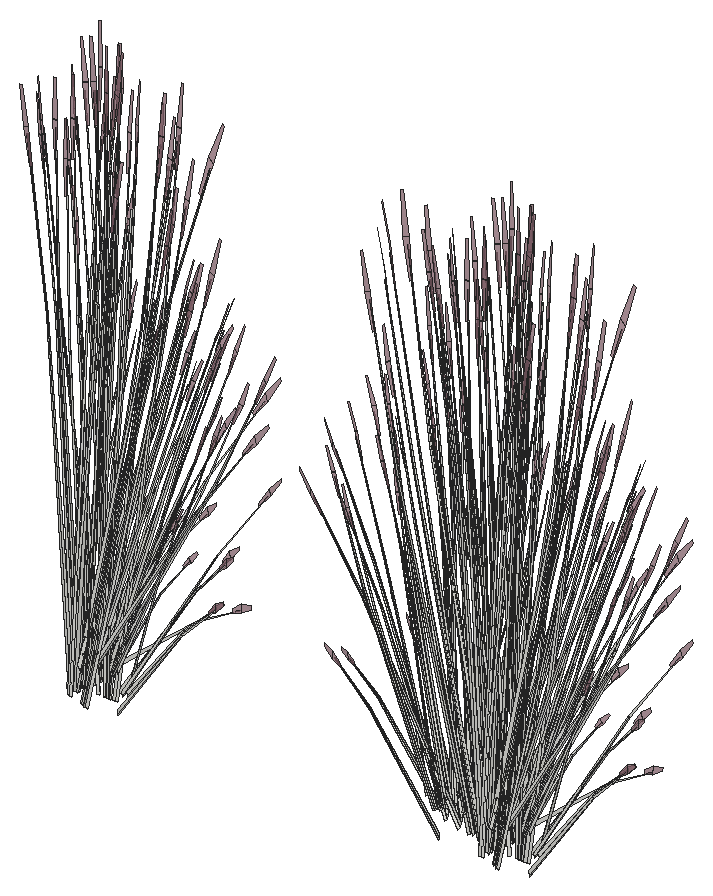
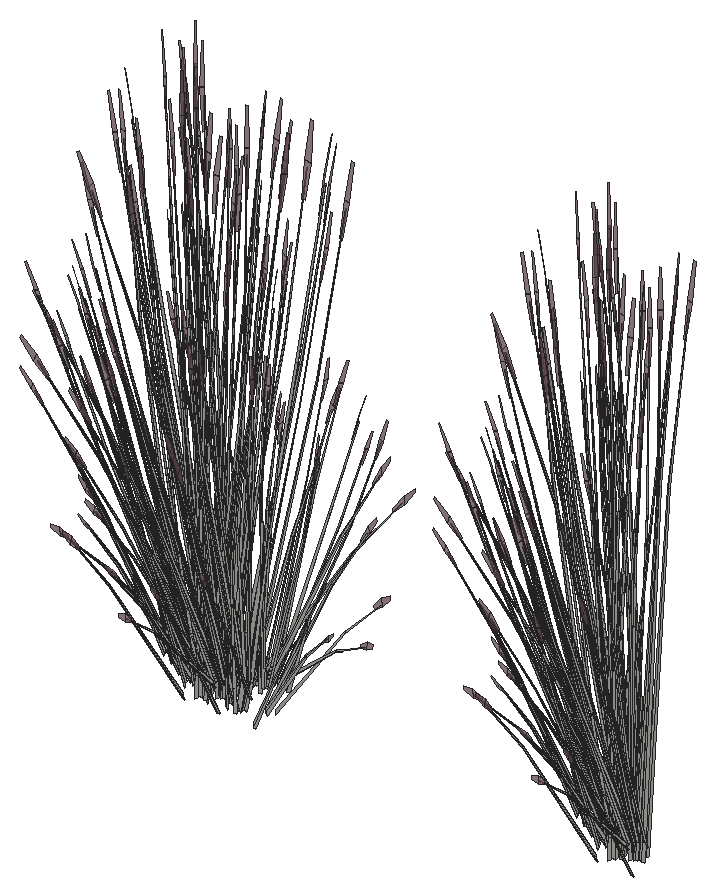
# SketchUp Ruby script. Lengths in inches.
U = 1.inch
M = Sketchup.active_model
def pt(a) = Geom::Point3d.new(a.map { |v| v * U })
def face(e, loops, mat)
  f = e.add_face(loops[0].map { |a| pt(a) })
  loops[1..].each { |l| e.add_face(l.map { |a| pt(a) }).erase! }
  f.material = f.back_material = mat if mat
  f
end
# faces: each face lists its corners as indices into pts; further lists are holes
def faces(e, pts, list, mat = nil) = list.each { |f| face(e, (f[0].is_a?(Array) ? f : [f]).map { |l| l.map { |i| pts[i] } }, mat) }
# xy, xz, yz: faces in a plane at the given z, y or x. An outline is a flat list of corners, or four numbers for a rectangle; further outlines are holes
def ring(l) = l.size == 4 ? [[l[0], l[1]], [l[2], l[1]], [l[2], l[3]], [l[0], l[3]]] : l.each_slice(2).to_a
def flat(e, list, mat, &to3) = list.each { |f| face(e, (f[0].is_a?(Array) ? f : [f]).map { |l| ring(l).map { |u, v| to3.(u, v) } }, mat) }
def xy(e, z, list, mat = nil) = flat(e, list, mat) { |x, y| [x, y, z] }
def xz(e, y, list, mat = nil) = flat(e, list, mat) { |x, z| [x, y, z] }
def yz(e, x, list, mat = nil) = flat(e, list, mat) { |y, z| [x, y, z] }
def lines(e, pts, list) = list.each { |a, b| e.add_line(pt(pts[a]), pt(pts[b])) }
# prism: a flat outline (further loops are holes) pulled along v
def prism(e, loops, v, mat = nil)
  f = face(e, loops, mat); d = Geom::Vector3d.new(v.map { |x| x * U })
  f.pushpull(f.normal.samedirection?(d) ? d.length : -d.length)
end
def box(e, o, s, mat = nil) = prism(e, [[o, [o[0] + s[0], o[1], o[2]], [o[0] + s[0], o[1] + s[1], o[2]], [o[0], o[1] + s[1], o[2]]]], [0, 0, s[2]], mat)
def at(x, y, z, deg = 0) = Geom::Transformation.translation(pt([x, y, z])) * Geom::Transformation.rotation(ORIGIN, Z_AXIS, deg.degrees)
def axes(o, x, y, z) = Geom::Transformation.new([*x, 0, *y, 0, *z, 0, *pt(o).to_a, 1])
def part(name) = M.definitions.add(name)
# library, detail: a bought-in or finely detailed component or shape, given as its bounding box
def library(name, o, s) = part(name).tap { |d| box(d.entities, o, s) }
def detail(e, o, s) = box(e.add_group.entities, o, s)
def put(e, d, t, mat = nil) = e.add_instance(d, t).tap { |i| i.material = mat if mat }
def group(e, t, mat = nil) = e.add_group.tap { |g| g.transformation = t; g.material = mat if mat }.entities
root = M.entities
M.materials.add("LightPink_Translucent").color = [144, 107, 117]
M.materials["LightPink_Translucent"].alpha = 0.75
c1 = part("blade")
p = [[2.15,0.21,22],[0,0.17,0],[0.09,0.45,0],[2.18,0.31,22],[2.29,0.31,22],[0.38,0.45,0],
  [2.48,0.24,33],[2.49,0.24,33],[2.48,0.22,33]]
faces(c1.entities,p,[[0,1,2,3],[4,5,2,3],[6,3,4,7],[8,0,3,6]])
c2 = part("seeds")
p = [[0.3,-0.1,1.38],[-0.01,-0.03,1.59],[-0.01,-0.03,0.03],[0.14,-0.07,-0.07],[0.29,-0.03,3],[0.15,0.01,3.11]]
faces(c2.entities,p,[[0,1,2,3],[1,0,4,5]],"LightPink_Translucent")
c3 = part("blade with seeds")
put(c3.entities,c1,at(0,0,0))
put(c3.entities,c2,axes([2.4,0.25,30.99],[1.5799,-0.05474,1.17369],[-0.12525,1.92788,0.29478],[-0.07173,-0.02425,1.56792]))
put(root,c3,axes([817.6,482.08,3.9375],[-0.01125,-0.12549,0.85688],[0.48751,0.08325,0.06928],[-0.03015,0.17883,0.36631]))
put(root,c3,axes([818.01,481.54,3.18],[0.58084,0.06889,0.22877],[-0.11821,0.38906,0.08977],[-0.08488,-0.03757,0.79428]))
put(root,c3,axes([817.7,482.16,3.24],[0.49383,-0.08678,0.08821],[0.12194,0.32295,0.17543],[-0.04404,-0.04705,0.80203]))
put(root,c3,axes([818.33,482.21,3.1],[-0.4633,-0.14679,0],[0.22297,-0.30501,0],[0,0,0.81353]))
put(root,c3,axes([819.41,482.58,3.1875],[0.28732,0.32763,0],[-0.4807,0.18271,-0.25804],[-0.10948,0.04161,0.81856]))
put(root,c3,axes([817.94,482.72,4.53],[-0.45283,-0.08548,0.26641],[0.15485,-0.28101,0.21967],[0.02721,0.11051,0.55128]))
put(root,c3,axes([817.82,482.74,4.37],[-0.33863,0.11112,0.03215],[-0.16575,-0.20263,0.2531],[0.0327,0.08932,0.38595]))
put(root,c3,axes([819.17,482.18,3.24],[0.13276,-0.32494,0.08821],[0.4858,0.09195,0.17543],[-0.08392,0.00158,0.80203]))
put(root,c3,axes([818.94,481.75,3.31],[0.33952,0.19644,0.0724],[-0.2832,0.22163,-0.20674],[-0.07883,0.02996,0.63372]))
put(root,c3,axes([818.94,481.6,3.36],[0.49904,-0.02018,0.2237],[0.04513,0.33504,-0.10766],[-0.08934,0.03396,0.71822]))
put(root,c3,axes([819.06,482.375,3.17],[0.57533,0.10627,0.15378],[-0.14394,0.37986,-0.18246],[-0.09522,0.04754,0.82443]))
put(root,c3,axes([819.3,482.35,3.24],[0.4301,-0.16348,0.24825],[0.25708,0.29314,0],[-0.09796,0.03723,0.78752]))
put(root,c3,axes([818.44,482.09,3.1],[-0.14994,-0.28188,0],[0.42817,-0.09871,0],[0,0,0.77185]))
put(root,c3,axes([817.89,482.68,2.75],[0.07437,-0.01779,0.88171],[0.44738,0.09793,-0.1347],[0.01308,0.11037,0.15018]))
put(root,c3,axes([817.99,482.78,4.26],[-0.13855,0.25143,-0.17707],[-0.4042,-0.07334,0.2286],[0.03706,0.10123,0.4374]))
put(root,c3,axes([819.04,481.53,3.11],[-0.22297,0.29461,-0.2237],[-0.4633,-0.14179,0.10766],[0,0.06791,0.71822]))
put(root,c3,axes([817.71,483.23,4.36],[0.05825,0.05265,0.87472],[0.47011,0.02068,-0.13834],[0.04727,0.11612,0.07015]))
put(root,c3,axes([819.93,481.35,3.24],[-0.36107,-0.23816,0.08821],[0.36387,-0.231,0.17543],[-0.03988,0.04864,0.80203]))
put(root,c3,axes([818.97,481.36,3.15],[0,0.37813,-0.02818],[-0.57465,0,0],[0,0.01188,0.89684]))
put(root,c3,axes([817.95,482.51,4.53],[0.13855,-0.25143,0.17707],[0.4042,0.07334,-0.2286],[0.03706,0.10123,0.4374]))
put(root,c3,axes([818.69,482.1,3.15],[0.1998,0.37562,-0.03006],[-0.5709,0.13162,0],[0.00698,0.01312,0.86086]))
put(root,c3,axes([818.04,482.55,4.49],[0.21934,0.26585,-0.35523],[-0.45151,0.14816,0.04287],[0.05129,0.12845,0.5025]))
put(root,c3,axes([820.34,481.6,3.1],[-0.57436,-0.00261,-0.02488],[0,-0.36542,0.24971],[-0.01805,0.08319,0.79176]))
put(root,c3,axes([819.21,480.5,3.24],[-0.49383,0.08678,0.08821],[-0.12194,-0.32295,0.17543],[0.04404,0.04705,0.80203]))
put(root,c3,axes([818.49,483.41,4.82],[0.31757,-0.18757,-0.03244],[0.29098,0.20543,-0.14708],[0.02049,0.05821,0.48512]))
put(root,c3,axes([819.06,481.44,3.11],[0.32079,0.21119,0],[-0.32079,0.21119,0],[0,0,0.84633]))
put(root,c3,axes([819.05,481.19,3.36],[0.22297,-0.29461,0.2237],[0.4633,0.14179,-0.10766],[0,0.06791,0.71822]))
put(root,c3,axes([818.86,482.22,3.1],[0.4633,0.14679,0],[-0.22297,0.30501,0],[0,0,0.87477]))
put(root,c3,axes([818.2,482.61,4.34],[0.45175,0.08196,-0.25549],[-0.15485,0.28101,-0.1979],[0.04142,0.11314,0.48886]))
put(root,c3,axes([817.8125,482.62,4.52],[0.44971,-0.15222,-0.0608],[0.221,0.27017,-0.33747],[0.05933,0.11385,0.51278]))
put(root,c3,axes([818.9,481.125,3.19],[-0.58084,-0.06889,0.24599],[0.11821,-0.38906,0.09653],[0.08488,0.03757,0.85407]))
put(root,c3,axes([820.22,481.66,3.01],[-0.32079,0.20399,-0.15489],[-0.32079,-0.20399,0.15489],[0,0.06571,0.69487]))
put(root,c3,axes([819.31,481.62,3.05],[0.16851,0.29936,-0.34606],[-0.4854,0.10781,-0.09083],[0.01863,0.10137,0.76386]))
put(root,c3,axes([819.07,481.3,3.1],[0.51416,0,0],[0,0.33849,0],[0,0,0.89203]))
put(root,c3,axes([818.57,480.92,3.36],[-0.27607,-0.27443,0.2237],[0.41817,-0.19325,-0.10766],[0.08934,0.03396,0.71822]))
put(root,c3,axes([819.25,481.26,3.31],[0.42817,-0.09535,0.0724],[0.14994,0.27228,-0.20674],[0,0.05992,0.63372]))
put(root,c3,axes([819.1,481.28,3.33],[0.51755,0.15601,-0.14548],[-0.2492,0.32927,-0.25001],[0.01626,0.08084,0.79854]))
put(root,c3,axes([820.22,481.36,3.24],[0,-0.32696,0.24825],[0.51416,0,0],[0,0.07447,0.78752]))
put(root,c3,axes([820.44,481.66,3.01],[0,0.32696,-0.24825],[-0.51416,0,0],[0,0.07447,0.78752]))
put(root,c3,axes([819.07,482.65,4.37],[-0.45708,0.07503,0.24001],[-0.07933,-0.29434,0.1979],[0.1075,0.08675,0.49665]))
put(root,c3,axes([818.98,482.71,4.37],[-0.20887,0.2077,0.03215],[-0.29744,-0.12092,0.2531],[0.09616,0.06659,0.38595]))
put(root,c3,axes([818.46,482.03,3.9375],[-0.10505,-0.10498,0.85688],[0.48542,-0.08838,0.06928],[0.10971,0.1648,0.36631]))
put(root,c3,axes([819,482.05,3.09],[0.48247,-0.11094,-0.09599],[0.16954,0.31956,0.00004],[0.05326,-0.01226,0.86949]))
put(root,c3,axes([818.92,482.47,4.53],[-0.07098,-0.26335,0.17707],[0.40574,-0.06954,-0.2286],[0.10898,0.07547,0.4374]))
put(root,c3,axes([819.01,481.1,3.11],[0.27607,0.27443,-0.2237],[-0.41817,0.19325,0.10766],[0.08934,0.03396,0.71822]))
put(root,c3,axes([819.19,480.96,4.24],[-0.39711,-0.16988,0.69141],[0.41931,-0.2645,0.29833],[0.12812,0.1594,0.66832]))
put(root,c3,axes([818.52,482.84,4.35],[0.00136,-0.03958,0.88692],[0.39383,-0.17464,-0.08381],[0.1368,0.06234,0.15695]))
put(root,c3,axes([819.79,482.34,3.38],[-0.25875,-0.09401,0.5743],[0.33411,-0.09552,0.42196],[0.09012,0.08091,0.12649]))
put(root,c3,axes([818.87,482.24,3.3],[0.00811,-0.10838,0.71501],[0.38755,-0.12106,-0.15377],[0.11964,0.12972,0.3057]))
put(root,c3,axes([819.77,480.49,3.01],[0.10795,0.28489,-0.15489],[-0.42874,0.0809,0.15489],[0.08643,0.03285,0.69487]))
put(root,c3,axes([820.57,481.41,3.1875],[0.57465,0,0],[0,0.36542,-0.25804],[0,0.08323,0.81856]))
put(root,c3,axes([818.72,480.94,3.33],[0.46399,-0.21707,-0.14548],[0.30855,0.30672,-0.25001],[0.11448,0.03115,0.79854]))
put(root,c3,axes([819.83,482.77,3.33],[-0.2947,-0.01025,0.5253],[0.19462,-0.21779,0.29003],[0.11642,0.07737,0.41205]))
put(root,c3,axes([818.88,482.61,4.52],[0.27385,-0.27986,-0.0608],[0.39658,0.16123,-0.33747],[0.13785,0.07907,0.51278]))
put(root,c3,axes([819.21,482.47,4.34],[0.45348,-0.07772,-0.25549],[0.07933,0.29434,-0.1979],[0.1218,0.08435,0.48886]))
put(root,c3,axes([819.73,482.12,4.53],[-0.26148,-0.20471,0.17707],[0.29857,-0.19378,-0.2286],[0.1517,0.02948,0.4374]))
put(root,c3,axes([819.89,480.36,3.01],[0.4301,0.16348,-0.24825],[-0.25708,0.29314,0],[0.09796,0.03723,0.78752]))
put(root,c3,axes([819.96,482.3,4.37],[-0.02314,0.24862,0.03215],[-0.34943,-0.00682,0.2531],[0.13385,0.02602,0.38595]))
put(root,c3,axes([819.86,482.69,2.75],[0.03348,-0.0472,0.88171],[0.42153,-0.13902,-0.1347],[0.12779,0.07195,0.15018]))
put(root,c3,axes([820,482.22,4.37],[-0.33886,0.21544,0.24001],[-0.29224,-0.22879,0.1979],[0.15898,0.03974,0.49665]))
put(root,c3,axes([820.875,482.26,3.96],[-0.08796,-0.27485,-0.01746],[0.41573,-0.06319,-0.07916],[0.08682,0.01742,0.26109]))
put(root,c3,axes([819.26,480.99,3.03],[0.47805,0.0536,-0.31177],[-0.10088,0.33065,-0.08182],[0.14266,0.04007,0.68817]))
put(root,c3,axes([819.16,481.7,3.9375],[-0.1707,-0.05633,0.85688],[0.35326,-0.23632,0.06928],[0.22018,0.10661,0.36631]))
put(root,c3,axes([820.5,481.625,4.37],[0.16879,0.22293,0.03215],[-0.30779,0.10912,0.2531],[0.13568,-0.02153,0.38595]))
put(root,c3,axes([820.1,482.22,4.26],[0.26148,0.20471,-0.17707],[-0.29857,0.19378,0.2286],[0.1517,0.02948,0.4374]))
put(root,c3,axes([819.8,482.25,4.52],[0.02461,-0.33251,-0.0608],[0.4659,0.00909,-0.33747],[0.17944,0.0231,0.51278]))
put(root,c3,axes([820.47,481.55,4.37],[-0.12984,0.29812,0.24001],[-0.42685,-0.10194,0.1979],[0.16786,-0.01792,0.49665]))
put(root,c3,axes([820.2,482.05,4.36],[0.09858,-0.00553,0.87472],[0.2704,-0.25401,-0.13834],[0.17535,0.03353,0.07015]))
put(root,c3,axes([821.37,481.57,3.38],[-0.28394,0.05398,0.5743],[0.13365,-0.22308,0.42196],[0.15063,0.01526,0.12649]))
put(root,c3,axes([820.56,481.51,4.26],[0.38192,0.09121,-0.17707],[-0.11139,0.2661,0.2286],[0.15377,-0.0244,0.4374]))
put(root,c3,axes([819.82,482.09,4.49],[0.45939,0.00787,-0.35523],[-0.03085,0.3315,0.04287],[0.19462,0.03498,0.5025]))
put(root,c3,axes([821.08,481.26,2.75],[-0.02402,-0.04964,0.88171],[0.16658,-0.29036,-0.1347],[0.16804,-0.00418,0.15018]))
put(root,c3,axes([821.24,482.51,4.35],[-0.04155,-0.02862,0.88692],[0.0909,-0.30682,-0.08381],[0.16368,-0.0196,0.15695]))
put(root,c3,axes([819.52,481.18,3.9375],[-0.19062,0.00741,0.85688],[0.12645,-0.32094,0.06928],[0.27165,0.01985,0.36631]))
put(root,c3,axes([820.84,481.93,3.3],[-0.11068,-0.08041,0.71501],[0.144,-0.26601,-0.15377],[0.22393,0.03604,0.3057]))
put(root,c3,axes([838.9,481.38,3.9375],[0.15946,-0.06916,0.85688],[0.13424,0.31957,0.06928],[-0.25033,0.07223,0.36631]))
put(root,c3,axes([838.41,481.92,3.3],[0.15971,0.02684,0.71501],[0.10294,0.27415,-0.15377],[-0.21694,0.05132,0.3057]))
put(root,c3,axes([839.82,481.05,3.67],[0.13063,-0.0473,0.88532],[0.04505,0.33024,0.06928],[-0.28294,0.04382,0.31642]))
put(root,c3,axes([838.42,481.27,4.36],[-0.07505,0.04245,0.87472],[0.00638,0.31015,-0.13834],[-0.17202,0.04033,0.07015]))
put(root,c3,axes([838.66,481.09,4.26],[-0.38192,-0.09121,-0.17707],[0.11139,-0.2661,0.2286],[-0.15377,0.0244,0.4374]))
put(root,c3,axes([837.58,481.58,4.35],[0.05865,0.00877,0.88692],[0.18143,0.28888,-0.08381],[-0.12006,0.07582,0.15695]))
put(root,c3,axes([838.92,481.23,4.34],[-0.1245,0.29741,-0.25549],[-0.42685,-0.10194,-0.1979],[-0.17186,0.02727,0.48886]))
put(root,c3,axes([838.7,481.21,2.75],[0.01165,0.05153,0.88171],[-0.23495,0.26909,-0.1347],[-0.16689,-0.01356,0.15018]))
put(root,c3,axes([838.07,482.5,3.38],[0.19152,-0.14818,0.5743],[0.07557,0.23459,0.42196],[-0.13841,0.042,0.12649]))
put(root,c3,axes([838.9,480.97,4.52],[0.23123,0.29606,-0.0608],[-0.41039,0.14549,-0.33747],[-0.17294,0.03906,0.51278]))
put(root,c3,axes([838.71,480.98,4.37],[-0.16879,-0.22293,0.03215],[0.30779,-0.10912,0.2531],[-0.13568,0.02153,0.38595]))
put(root,c3,axes([839.49,481.59,3.9375],[0.11478,-0.10046,0.85688],[0.28982,0.27117,0.06928],[-0.19878,0.12349,0.36631]))
put(root,c3,axes([838.8,481.86,4.26],[-0.40003,0.04673,-0.17707],[-0.10563,-0.26712,0.2286],[-0.11464,0.07175,0.4374]))
put(root,c3,axes([838.58,482.65,2.75],[0.06164,0.03267,0.88171],[0.10452,0.30266,-0.1347],[-0.13662,0.06454,0.15018]))
put(root,c3,axes([838.85,481.8,4.37],[-0.11397,-0.30091,0.24001],[0.44709,-0.05222,0.1979],[-0.13177,0.07077,0.49665]))
put(root,c3,axes([838.76,481.74,4.37],[-0.31549,-0.13751,0.03215],[0.18368,-0.19581,0.2531],[-0.10115,0.06331,0.38595]))
put(root,c3,axes([839.4,481.84,3.9375],[0.08557,-0.11238,0.85688],[0.35897,0.23257,0.06928],[-0.16194,0.14495,0.36631]))
put(root,c3,axes([839.06,481.06,4.53],[0.38192,0.09121,0.17707],[-0.11139,0.2661,-0.2286],[-0.15377,0.0244,0.4374]))
put(root,c3,axes([839.125,481.89,4.34],[0.11806,0.29854,-0.25549],[-0.44709,0.05222,-0.1979],[-0.12812,0.08019,0.48886]))
put(root,c3,axes([838.43,482.42,4.36],[-0.01142,0.0647,0.87472],[0.32418,0.22509,-0.13834],[-0.08487,0.10644,0.07015]))
put(root,c3,axes([839.61,482.3,3.01],[-0.4301,-0.16348,-0.24825],[0.25708,-0.29314,0],[-0.09796,-0.03723,0.78752]))
put(root,c3,axes([838.92,481.67,4.52],[0.4251,0.18028,-0.0608],[-0.24491,0.26108,-0.33747],[-0.1201,0.09075,0.51278]))
put(root,c3,axes([839.875,482.5,3.1875],[-0.28732,0.32763,0],[-0.4807,-0.18271,-0.25804],[-0.10948,-0.04161,0.81856]))
put(root,c3,axes([838.22,482.46,4.82],[0.40553,0.08728,-0.03244],[-0.12475,0.26862,-0.14708],[-0.06633,0.04078,0.48512]))
put(root,c3,axes([839.125,481.7,4.53],[0.40003,-0.04673,0.17707],[0.10563,0.26712,-0.2286],[-0.11464,0.07175,0.4374]))
put(root,c3,axes([839.35,482.97,3.3],[0.14502,-0.05158,0.71501],[0.35805,0.15552,-0.15377],[-0.10657,0.13457,0.3057]))
put(root,c3,axes([840.78,481.72,3.33],[-0.46399,0.21707,-0.14548],[-0.30855,-0.30672,-0.25001],[-0.11448,-0.03115,0.79854]))
put(root,c3,axes([839.5,482.41,4.37],[-0.32725,-0.22308,0.24001],[0.34753,-0.1924,0.1979],[-0.06036,0.10466,0.49665]))
put(root,c3,axes([839.73,482.18,3.01],[-0.10795,-0.28489,-0.15489],[0.42874,-0.0809,0.15489],[-0.08643,-0.03285,0.69487]))
put(root,c3,axes([839.38,482.39,4.37],[-0.37765,-0.01523,0.03215],[0.01035,-0.23004,0.2531],[-0.03952,0.08812,0.38595]))
put(root,c3,axes([839.5,482.48,4.26],[-0.31095,0.17214,-0.17707],[-0.29435,-0.19656,0.2286],[-0.04479,0.09987,0.4374]))
put(root,c3,axes([841.09,481.96,3.03],[-0.30954,0.24575,-0.31177],[-0.38452,-0.22284,-0.08182],[-0.12404,0.0613,0.68817]))
put(root,c3,axes([838.39,483.09,4.35],[0.05214,-0.01974,0.88692],[0.43092,0.1313,-0.08381],[-0.01013,0.10932,0.15695]))
put(root,c3,axes([841.3,481.82,3.23],[-0.44875,-0.26316,-0.12596],[0.3776,-0.2955,0.27565],[-0.12084,0.03078,0.84108]))
put(root,c3,axes([839.71,482.29,4.67],[-0.01196,0.30243,-0.3943],[-0.50354,-0.02031,0.04758],[-0.05314,0.12813,0.55778]))
put(root,c3,axes([839.7,483.14,3.38],[-0.01189,-0.19441,0.5743],[0.29719,0.13866,0.42196],[-0.05845,0.09266,0.12649]))
put(root,c3,axes([841.08,481.77,3.11],[-0.49904,0.02018,-0.2237],[-0.04513,-0.33504,0.10766],[-0.08934,0.03396,0.71822]))
put(root,c3,axes([840.125,482.33,3.24],[0.4301,0.16348,0.24825],[-0.25708,0.29314,0],[-0.09796,-0.03723,0.78752]))
put(root,c3,axes([839.54,482.72,3.68],[0.0101,-0.16879,0.77173],[0.45413,0.08915,0.10664],[-0.03935,0.17989,0.36441]))
put(root,c3,axes([840.74,481.82,3.31],[-0.08866,0.29179,0.0724],[-0.43315,-0.05065,-0.20674],[-0.07883,-0.02996,0.63372]))
put(root,c3,axes([841.6,482.63,3.01],[-0.4301,0.16348,-0.24825],[-0.25708,-0.29314,0],[-0.09796,0.03723,0.78752]))
put(root,c3,axes([841.63,482.54,3.1],[-0.28374,-0.32877,-0.02571],[0.4807,-0.18271,0.25804],[-0.11845,0.0313,0.81815]))
put(root,c3,axes([839.81,482.39,4.5],[0.32898,0.21969,-0.2836],[-0.34753,0.1924,-0.21967],[-0.05006,0.11162,0.54264]))
put(root,c3,axes([841.5,482.5,3.01],[-0.42874,-0.0809,-0.15489],[0.10795,-0.28489,0.15489],[-0.08643,0.03285,0.69487]))
put(root,c3,axes([839.66,482.23,4.53],[0.31095,-0.17214,0.17707],[0.29435,0.19656,-0.2286],[-0.04479,0.09987,0.4374]))
put(root,c3,axes([841.75,481.28,3.42],[-0.01255,-0.30784,0.70636],[0.56816,0.0798,0.29908],[-0.13438,0.16845,0.66675]))
put(root,c3,axes([839.47,482.28,4.7],[0.50507,0.0162,-0.06749],[-0.01381,0.30672,-0.3746],[-0.03508,0.11813,0.56919]))
put(root,c3,axes([839.45,482.72,3.41],[0.41748,-0.0579,0.03254],[0.09598,0.23326,-0.43152],[-0.02647,0.11808,0.3868]))
put(root,c3,axes([841.43,481.68,3.33],[0.05355,0.37308,-0.14548],[-0.55775,0.02256,-0.25001],[-0.09822,0.04969,0.79854]))
put(root,c3,axes([840.18,482.08,3.9375],[-0.01125,-0.12549,0.85688],[0.48751,0.08325,0.06928],[-0.03015,0.17883,0.36631]))
put(root,c3,axes([840.6,481.54,3.18],[0.58084,0.06889,0.22877],[-0.11821,0.38906,0.08977],[-0.08488,-0.03757,0.79428]))
put(root,c3,axes([840.28,482.16,3.24],[0.49383,-0.08678,0.08821],[0.12194,0.32295,0.17543],[-0.04404,-0.04705,0.80203]))
put(root,c3,axes([840.92,482.21,3.1],[-0.4633,-0.14679,0],[0.22297,-0.30501,0],[0,0,0.81353]))
put(root,c3,axes([841.99,482.58,3.1875],[0.28732,0.32763,0],[-0.4807,0.18271,-0.25804],[-0.10948,0.04161,0.81856]))
put(root,c3,axes([840.53,482.72,4.53],[-0.45283,-0.08548,0.26641],[0.15485,-0.28101,0.21967],[0.02721,0.11051,0.55128]))
put(root,c3,axes([840.41,482.74,4.37],[-0.33863,0.11112,0.03215],[-0.16575,-0.20263,0.2531],[0.0327,0.08932,0.38595]))
put(root,c3,axes([841.75,482.18,3.24],[0.13276,-0.32494,0.08821],[0.4858,0.09195,0.17543],[-0.08392,0.00158,0.80203]))
put(root,c3,axes([841.53,481.75,3.31],[0.33952,0.19644,0.0724],[-0.2832,0.22163,-0.20674],[-0.07883,0.02996,0.63372]))
put(root,c3,axes([841.52,481.6,3.36],[0.49904,-0.02018,0.2237],[0.04513,0.33504,-0.10766],[-0.08934,0.03396,0.71822]))
put(root,c3,axes([841.64,482.375,3.17],[0.57533,0.10627,0.15378],[-0.14394,0.37986,-0.18246],[-0.09522,0.04754,0.82443]))
put(root,c3,axes([841.89,482.35,3.24],[0.4301,-0.16348,0.24825],[0.25708,0.29314,0],[-0.09796,0.03723,0.78752]))
put(root,c3,axes([841.03,482.09,3.1],[-0.14994,-0.28188,0],[0.42817,-0.09871,0],[0,0,0.77185]))
put(root,c3,axes([840.48,482.68,2.75],[0.07437,-0.01779,0.88171],[0.44738,0.09793,-0.1347],[0.01308,0.11037,0.15018]))
put(root,c3,axes([840.58,482.78,4.26],[-0.13855,0.25143,-0.17707],[-0.4042,-0.07334,0.2286],[0.03706,0.10123,0.4374]))
put(root,c3,axes([841.63,481.53,3.11],[-0.22297,0.29461,-0.2237],[-0.4633,-0.14179,0.10766],[0,0.06791,0.71822]))
put(root,c3,axes([840.29,483.23,4.36],[0.05825,0.05265,0.87472],[0.47011,0.02068,-0.13834],[0.04727,0.11612,0.07015]))
put(root,c3,axes([842.51,481.35,3.24],[-0.36107,-0.23816,0.08821],[0.36387,-0.231,0.17543],[-0.03988,0.04864,0.80203]))
put(root,c3,axes([841.55,481.36,3.15],[0,0.37813,-0.02818],[-0.57465,0,0],[0,0.01188,0.89684]))
put(root,c3,axes([840.54,482.51,4.53],[0.13855,-0.25143,0.17707],[0.4042,0.07334,-0.2286],[0.03706,0.10123,0.4374]))
put(root,c3,axes([841.28,482.1,3.15],[0.1998,0.37562,-0.03006],[-0.5709,0.13162,0],[0.00698,0.01312,0.86086]))
put(root,c3,axes([840.62,482.55,4.49],[0.21934,0.26585,-0.35523],[-0.45151,0.14816,0.04287],[0.05129,0.12845,0.5025]))
put(root,c3,axes([842.93,481.6,3.1],[-0.57436,-0.00261,-0.02488],[0,-0.36542,0.24971],[-0.01805,0.08319,0.79176]))
put(root,c3,axes([841.8,480.5,3.24],[-0.49383,0.08678,0.08821],[-0.12194,-0.32295,0.17543],[0.04404,0.04705,0.80203]))
put(root,c3,axes([841.08,483.41,4.82],[0.31757,-0.18757,-0.03244],[0.29098,0.20543,-0.14708],[0.02049,0.05821,0.48512]))
put(root,c3,axes([841.64,481.44,3.11],[0.32079,0.21119,0],[-0.32079,0.21119,0],[0,0,0.84633]))
put(root,c3,axes([841.64,481.19,3.36],[0.22297,-0.29461,0.2237],[0.4633,0.14179,-0.10766],[0,0.06791,0.71822]))
put(root,c3,axes([841.45,482.22,3.1],[0.4633,0.14679,0],[-0.22297,0.30501,0],[0,0,0.87477]))
put(root,c3,axes([840.79,482.61,4.34],[0.45175,0.08196,-0.25549],[-0.15485,0.28101,-0.1979],[0.04142,0.11314,0.48886]))
put(root,c3,axes([840.4,482.62,4.52],[0.44971,-0.15222,-0.0608],[0.221,0.27017,-0.33747],[0.05933,0.11385,0.51278]))
put(root,c3,axes([841.49,481.125,3.19],[-0.58084,-0.06889,0.24599],[0.11821,-0.38906,0.09653],[0.08488,0.03757,0.85407]))
put(root,c3,axes([842.81,481.66,3.01],[-0.32079,0.20399,-0.15489],[-0.32079,-0.20399,0.15489],[0,0.06571,0.69487]))
put(root,c3,axes([841.89,481.62,3.05],[0.16851,0.29936,-0.34606],[-0.4854,0.10781,-0.09083],[0.01863,0.10137,0.76386]))
put(root,c3,axes([841.66,481.3,3.1],[0.51416,0,0],[0,0.33849,0],[0,0,0.89203]))
put(root,c3,axes([841.16,480.92,3.36],[-0.27607,-0.27443,0.2237],[0.41817,-0.19325,-0.10766],[0.08934,0.03396,0.71822]))
put(root,c3,axes([841.83,481.26,3.31],[0.42817,-0.09535,0.0724],[0.14994,0.27228,-0.20674],[0,0.05992,0.63372]))
put(root,c3,axes([841.6875,481.28,3.33],[0.51755,0.15601,-0.14548],[-0.2492,0.32927,-0.25001],[0.01626,0.08084,0.79854]))
put(root,c3,axes([842.81,481.36,3.24],[0,-0.32696,0.24825],[0.51416,0,0],[0,0.07447,0.78752]))
put(root,c3,axes([843.03,481.66,3.01],[0,0.32696,-0.24825],[-0.51416,0,0],[0,0.07447,0.78752]))
put(root,c3,axes([841.66,482.65,4.37],[-0.45708,0.07503,0.24001],[-0.07933,-0.29434,0.1979],[0.1075,0.08675,0.49665]))
put(root,c3,axes([841.57,482.71,4.37],[-0.20887,0.2077,0.03215],[-0.29744,-0.12092,0.2531],[0.09616,0.06659,0.38595]))
put(root,c3,axes([841.04,482.03,3.9375],[-0.10505,-0.10498,0.85688],[0.48542,-0.08838,0.06928],[0.10971,0.1648,0.36631]))
put(root,c3,axes([841.59,482.05,3.09],[0.48247,-0.11094,-0.09599],[0.16954,0.31956,0.00004],[0.05326,-0.01226,0.86949]))
put(root,c3,axes([841.51,482.47,4.53],[-0.07098,-0.26335,0.17707],[0.40574,-0.06954,-0.2286],[0.10898,0.07547,0.4374]))
put(root,c3,axes([841.6,481.1,3.11],[0.27607,0.27443,-0.2237],[-0.41817,0.19325,0.10766],[0.08934,0.03396,0.71822]))
put(root,c3,axes([841.78,480.96,4.24],[-0.39711,-0.16988,0.69141],[0.41931,-0.2645,0.29833],[0.12812,0.1594,0.66832]))
put(root,c3,axes([841.11,482.84,4.35],[0.00136,-0.03958,0.88692],[0.39383,-0.17464,-0.08381],[0.1368,0.06234,0.15695]))
put(root,c3,axes([842.38,482.34,3.38],[-0.25875,-0.09401,0.5743],[0.33411,-0.09552,0.42196],[0.09012,0.08091,0.12649]))
put(root,c3,axes([841.46,482.24,3.3],[0.00811,-0.10838,0.71501],[0.38755,-0.12106,-0.15377],[0.11964,0.12972,0.3057]))
put(root,c3,axes([842.35,480.49,3.01],[0.10795,0.28489,-0.15489],[-0.42874,0.0809,0.15489],[0.08643,0.03285,0.69487]))
put(root,c3,axes([843.16,481.41,3.1875],[0.57465,0,0],[0,0.36542,-0.25804],[0,0.08323,0.81856]))
put(root,c3,axes([841.3,480.94,3.33],[0.46399,-0.21707,-0.14548],[0.30855,0.30672,-0.25001],[0.11448,0.03115,0.79854]))
put(root,c3,axes([842.42,482.77,3.33],[-0.2947,-0.01025,0.5253],[0.19462,-0.21779,0.29003],[0.11642,0.07737,0.41205]))
put(root,c3,axes([841.47,482.61,4.52],[0.27385,-0.27986,-0.0608],[0.39658,0.16123,-0.33747],[0.13785,0.07907,0.51278]))
put(root,c3,axes([841.79,482.47,4.34],[0.45348,-0.07772,-0.25549],[0.07933,0.29434,-0.1979],[0.1218,0.08435,0.48886]))
put(root,c3,axes([842.3125,482.12,4.53],[-0.26148,-0.20471,0.17707],[0.29857,-0.19378,-0.2286],[0.1517,0.02948,0.4374]))
put(root,c3,axes([842.47,480.36,3.01],[0.4301,0.16348,-0.24825],[-0.25708,0.29314,0],[0.09796,0.03723,0.78752]))
put(root,c3,axes([842.55,482.3,4.37],[-0.02314,0.24862,0.03215],[-0.34943,-0.00682,0.2531],[0.13385,0.02602,0.38595]))
put(root,c3,axes([842.45,482.69,2.75],[0.03348,-0.0472,0.88171],[0.42153,-0.13902,-0.1347],[0.12779,0.07195,0.15018]))
put(root,c3,axes([842.58,482.22,4.37],[-0.33886,0.21544,0.24001],[-0.29224,-0.22879,0.1979],[0.15898,0.03974,0.49665]))
put(root,c3,axes([843.46,482.26,3.96],[-0.08796,-0.27485,-0.01746],[0.41573,-0.06319,-0.07916],[0.08682,0.01742,0.26109]))
put(root,c3,axes([841.84,480.99,3.03],[0.47805,0.0536,-0.31177],[-0.10088,0.33065,-0.08182],[0.14266,0.04007,0.68817]))
put(root,c3,axes([841.75,481.7,3.9375],[-0.1707,-0.05633,0.85688],[0.35326,-0.23632,0.06928],[0.22018,0.10661,0.36631]))
put(root,c3,axes([843.09,481.625,4.37],[0.16879,0.22293,0.03215],[-0.30779,0.10912,0.2531],[0.13568,-0.02153,0.38595]))
put(root,c3,axes([842.68,482.22,4.26],[0.26148,0.20471,-0.17707],[-0.29857,0.19378,0.2286],[0.1517,0.02948,0.4374]))
put(root,c3,axes([842.39,482.25,4.52],[0.02461,-0.33251,-0.0608],[0.4659,0.00909,-0.33747],[0.17944,0.0231,0.51278]))
put(root,c3,axes([843.06,481.55,4.37],[-0.12984,0.29812,0.24001],[-0.42685,-0.10194,0.1979],[0.16786,-0.01792,0.49665]))
put(root,c3,axes([842.79,482.05,4.36],[0.09858,-0.00553,0.87472],[0.2704,-0.25401,-0.13834],[0.17535,0.03353,0.07015]))
put(root,c3,axes([843.96,481.57,3.38],[-0.28394,0.05398,0.5743],[0.13365,-0.22308,0.42196],[0.15063,0.01526,0.12649]))
put(root,c3,axes([843.15,481.51,4.26],[0.38192,0.09121,-0.17707],[-0.11139,0.2661,0.2286],[0.15377,-0.0244,0.4374]))
put(root,c3,axes([842.41,482.09,4.49],[0.45939,0.00787,-0.35523],[-0.03085,0.3315,0.04287],[0.19462,0.03498,0.5025]))
put(root,c3,axes([843.66,481.26,2.75],[-0.02402,-0.04964,0.88171],[0.16658,-0.29036,-0.1347],[0.16804,-0.00418,0.15018]))
put(root,c3,axes([843.82,482.51,4.35],[-0.04155,-0.02862,0.88692],[0.0909,-0.30682,-0.08381],[0.16368,-0.0196,0.15695]))
put(root,c3,axes([842.11,481.18,3.9375],[-0.19062,0.00741,0.85688],[0.12645,-0.32094,0.06928],[0.27165,0.01985,0.36631]))
put(root,c3,axes([843.42,481.93,3.3],[-0.11068,-0.08041,0.71501],[0.144,-0.26601,-0.15377],[0.22393,0.03604,0.3057]))
